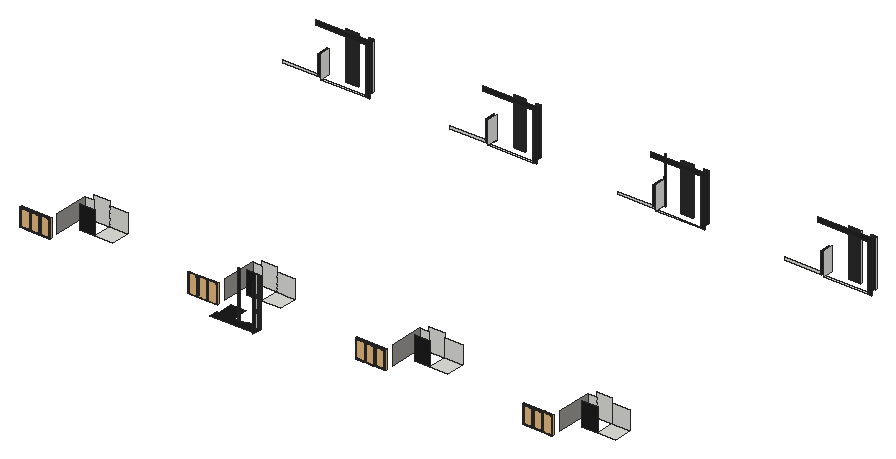
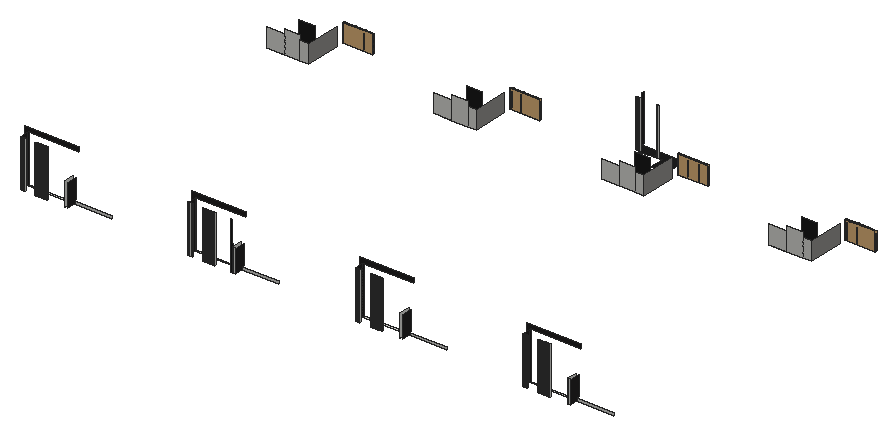
# SketchUp Ruby script. Lengths in inches.
U = 1.inch
M = Sketchup.active_model
def pt(a) = Geom::Point3d.new(a.map { |v| v * U })
def face(e, loops, mat)
  f = e.add_face(loops[0].map { |a| pt(a) })
  loops[1..].each { |l| e.add_face(l.map { |a| pt(a) }).erase! }
  f.material = f.back_material = mat if mat
  f
end
# faces: each face lists its corners as indices into pts; further lists are holes
def faces(e, pts, list, mat = nil) = list.each { |f| face(e, (f[0].is_a?(Array) ? f : [f]).map { |l| l.map { |i| pts[i] } }, mat) }
# xy, xz, yz: faces in a plane at the given z, y or x. An outline is a flat list of corners, or four numbers for a rectangle; further outlines are holes
def ring(l) = l.size == 4 ? [[l[0], l[1]], [l[2], l[1]], [l[2], l[3]], [l[0], l[3]]] : l.each_slice(2).to_a
def flat(e, list, mat, &to3) = list.each { |f| face(e, (f[0].is_a?(Array) ? f : [f]).map { |l| ring(l).map { |u, v| to3.(u, v) } }, mat) }
def xy(e, z, list, mat = nil) = flat(e, list, mat) { |x, y| [x, y, z] }
def xz(e, y, list, mat = nil) = flat(e, list, mat) { |x, z| [x, y, z] }
def yz(e, x, list, mat = nil) = flat(e, list, mat) { |y, z| [x, y, z] }
def lines(e, pts, list) = list.each { |a, b| e.add_line(pt(pts[a]), pt(pts[b])) }
# prism: a flat outline (further loops are holes) pulled along v
def prism(e, loops, v, mat = nil)
  f = face(e, loops, mat); d = Geom::Vector3d.new(v.map { |x| x * U })
  f.pushpull(f.normal.samedirection?(d) ? d.length : -d.length)
end
def box(e, o, s, mat = nil) = prism(e, [[o, [o[0] + s[0], o[1], o[2]], [o[0] + s[0], o[1] + s[1], o[2]], [o[0], o[1] + s[1], o[2]]]], [0, 0, s[2]], mat)
def at(x, y, z, deg = 0) = Geom::Transformation.translation(pt([x, y, z])) * Geom::Transformation.rotation(ORIGIN, Z_AXIS, deg.degrees)
def axes(o, x, y, z) = Geom::Transformation.new([*x, 0, *y, 0, *z, 0, *pt(o).to_a, 1])
def part(name) = M.definitions.add(name)
# library, detail: a bought-in or finely detailed component or shape, given as its bounding box
def library(name, o, s) = part(name).tap { |d| box(d.entities, o, s) }
def detail(e, o, s) = box(e.add_group.entities, o, s)
def put(e, d, t, mat = nil) = e.add_instance(d, t).tap { |i| i.material = mat if mat }
def group(e, t, mat = nil) = e.add_group.tap { |g| g.transformation = t; g.material = mat if mat }.entities
root = M.entities
M.materials.add("Wine2").color = [0, 0, 0]
M.materials["Wine2"].alpha = 0
M.materials.add("[0130_Gainsboro]").color = [39, 45, 50]
M.materials.add("[Color M08]").color = [30, 30, 30]
M.materials.add("[Field Square Tile]").color = [211, 167, 108]
M.materials.add("[Granite Dark Gray]").color = [38, 37, 37]
M.materials.add("[Granite Light Gray]").color = [149, 148, 144]
M.materials.add("[Slate]").color = [102, 110, 108]
c1 = part("Group\#55")
xy(c1.entities,0,[[0,-0.98,43.07,0],[0,0,43.07,1.4]],"[0130_Gainsboro]")
xy(c1.entities,0.3,[[0.3,-1.43,42.77,-0.98]],"[0130_Gainsboro]")
xy(c1.entities,2.95,[[2.95,-1.43,40.12,-0.63],[2.95,-0.63,40.12,0],[2.95,0,40.12,0.64],[2.95,0.64,40.12,1.4]],"[0130_Gainsboro]")
xy(c1.entities,3.54,[[3.54,-0.63,39.53,0],[3.54,0,39.53,0.64]],"[0130_Gainsboro]")
xy(c1.entities,111.8125,[[3.54,-0.63,39.53,0],[3.54,0,39.53,0.64]],"[0130_Gainsboro]")
xy(c1.entities,112.4,[[2.95,-1.43,40.12,-0.63],[2.95,-0.63,40.12,0],[2.95,0,40.12,0.64],[2.95,0.64,40.12,1.4]],"[0130_Gainsboro]")
xy(c1.entities,115.05,[[0.3,-1.43,42.77,-0.98]],"[0130_Gainsboro]")
xy(c1.entities,115.35,[[0,-0.98,43.07,0],[0,0,43.07,1.4]],"[0130_Gainsboro]")
xz(c1.entities,-1.43,[[[0.3,0.3,42.77,115.05],[2.95,2.95,40.12,112.4]]],"[0130_Gainsboro]")
xz(c1.entities,-0.98,[[[0,0,43.07,115.35],[0.3,0.3,42.77,115.05]]],"[0130_Gainsboro]")
xz(c1.entities,-0.63,[[[2.95,2.95,40.12,112.4],[3.54,3.54,39.53,111.8125]]],"[0130_Gainsboro]")
xz(c1.entities,0,[[3.54,3.54,39.53,111.8125]],"Wine2")
xz(c1.entities,0,[[[0,0,43.07,115.35],[2.95,2.95,40.12,112.4]],[[2.95,2.95,40.12,112.4],[3.54,3.54,39.53,111.8125]]],"[0130_Gainsboro]")
xz(c1.entities,0.64,[[[2.95,2.95,40.12,112.4],[3.54,3.54,39.53,111.8125]]],"[0130_Gainsboro]")
xz(c1.entities,1.4,[[[0,0,43.07,115.35],[2.95,2.95,40.12,112.4]]],"[0130_Gainsboro]")
yz(c1.entities,0,[[-0.98,0,0,115.35],[0,0,1.4,115.35]],"[0130_Gainsboro]")
yz(c1.entities,0.3,[[-1.43,0.3,-0.98,115.05]],"[0130_Gainsboro]")
yz(c1.entities,2.95,[[-1.43,2.95,-0.63,112.4],[-0.63,2.95,0,112.4],[0,2.95,0.64,112.4],[0.64,2.95,1.4,112.4]],"[0130_Gainsboro]")
yz(c1.entities,3.54,[[-0.63,3.54,0,111.8125],[0,3.54,0.64,111.8125]],"[0130_Gainsboro]")
yz(c1.entities,39.53,[[-0.63,3.54,0,111.8125],[0,3.54,0.64,111.8125]],"[0130_Gainsboro]")
yz(c1.entities,40.12,[[-1.43,2.95,-0.63,112.4],[-0.63,2.95,0,112.4],[0,2.95,0.64,112.4],[0.64,2.95,1.4,112.4]],"[0130_Gainsboro]")
yz(c1.entities,42.77,[[-1.43,0.3,-0.98,115.05]],"[0130_Gainsboro]")
yz(c1.entities,43.07,[[-0.98,0,0,115.35],[0,0,1.4,115.35]],"[0130_Gainsboro]")
c2 = part("Component\#21")
put(c2.entities,c1,axes([90.57,1.43,0],[1.05148,0,0],[0,1,0],[0,0,1]))
put(c2.entities,c1,axes([0,1.43,0],[1.05148,0,0],[0,1,0],[0,0,1]))
put(c2.entities,c1,axes([45.29,1.43,0],[1.05148,0,0],[0,1,0],[0,0,1]))
c3 = library("Curtains",[0,0,0],[121.73,8.19,117.22])
xy(root,134.5,[[1452.96,508.33,1458.38,511.08],[1551.31,508.33,1555.29,511.08],[534.46,697.21,629.77,792.52],[1413.21,697.21,1508.52,792.52],[2291.96,697.21,2387.27,792.52],
  [3170.71,697.21,3266.02,792.52],[442.35,2294.125,676.54,2294.125,676.54,2303.93,444.78,2303.93,444.78,2346.71,442.35,2346.71],[1321.1,2294.125,1555.29,2294.125,1555.29,2303.93,1323.53,2303.93,1323.53,2346.71,1321.1,2346.71],[2199.85,2294.125,2434.04,2294.125,2434.04,2303.93,2202.28,2303.93,2202.28,2346.71,2199.85,2346.71],[3078.6,2294.125,3312.79,2294.125,3312.79,2303.93,3081.03,2303.93,3081.03,2346.71,3078.6,2346.71],
  [534.46,2343.96,539.88,2346.71],[541.08,2343.96,546.51,2346.71],[547.71,2343.96,553.13,2346.71],[554.33,2343.96,559.76,2346.71],[560.96,2343.96,566.38,2346.71],
  [567.58,2343.96,573.01,2346.71],[574.21,2343.96,579.63,2346.71],[580.83,2343.96,586.26,2346.71],[587.46,2343.96,592.88,2346.71],[594.08,2343.96,599.51,2346.71],
  [653.06,2343.96,658.48,2346.71],[659.68,2343.96,665.11,2346.71],[666.31,2343.96,671.73,2346.71],[672.56,2343.96,676.54,2346.71],[676.54,2343.96,677.98,2346.71],
  [1413.21,2343.96,1418.63,2346.71],[1419.83,2343.96,1425.26,2346.71],[1426.46,2343.96,1431.88,2346.71],[1433.08,2343.96,1438.51,2346.71],[1439.71,2343.96,1445.13,2346.71],
  [1446.33,2343.96,1451.76,2346.71],[1452.96,2343.96,1458.38,2346.71],[1459.58,2343.96,1465.01,2346.71],[1466.21,2343.96,1471.63,2346.71],[1472.83,2343.96,1478.26,2346.71],
  [1531.81,2343.96,1537.23,2346.71],[1538.43,2343.96,1543.86,2346.71],[1545.06,2343.96,1550.48,2346.71],[1551.31,2343.96,1555.29,2346.71],[1555.29,2343.96,1556.73,2346.71],
  [2291.96,2343.96,2297.38,2346.71],[2298.58,2343.96,2304.01,2346.71],[2305.21,2343.96,2310.63,2346.71],[2311.83,2343.96,2317.26,2346.71],[2318.46,2343.96,2323.88,2346.71],
  [2325.08,2343.96,2330.51,2346.71],[2331.71,2343.96,2337.13,2346.71],[2338.33,2343.96,2343.76,2346.71],[2344.96,2343.96,2350.38,2346.71],[2351.58,2343.96,2357.01,2346.71],
  [2410.56,2343.96,2415.98,2346.71],[2417.18,2343.96,2422.61,2346.71],[2423.81,2343.96,2429.23,2346.71],[2430.06,2343.96,2434.04,2346.71],[2434.04,2343.96,2435.48,2346.71],
  [3170.71,2343.96,3176.13,2346.71],[3177.33,2343.96,3182.76,2346.71],[3183.96,2343.96,3189.38,2346.71],[3190.58,2343.96,3196.01,2346.71],[3197.21,2343.96,3202.63,2346.71],
  [3203.83,2343.96,3209.26,2346.71],[3210.46,2343.96,3215.88,2346.71],[3217.08,2343.96,3222.51,2346.71],[3223.71,2343.96,3229.13,2346.71],[3230.33,2343.96,3235.76,2346.71],
  [3289.31,2343.96,3294.73,2346.71],[3295.93,2343.96,3301.36,2346.71],[3302.56,2343.96,3307.98,2346.71],[3308.81,2343.96,3312.79,2346.71],[3312.79,2343.96,3314.23,2346.71]])
xy(root,134.5,[[1323.53,468.31,1555.29,468.31,1555.29,508.33,1551.31,508.33,1551.31,511.08,1550.48,511.08,1550.48,508.33,1545.06,508.33,1545.06,511.08,1543.86,511.08,1543.86,508.33,1538.43,508.33,1538.43,511.08,1537.23,511.08,1537.23,508.33,1531.81,508.33,1531.81,518.65,1483.9375,518.65,1483.9375,513.52,1478.26,513.52,1478.26,508.33,1472.83,508.33,1472.83,511.08,1471.63,511.08,1471.63,508.33,1466.21,508.33,1466.21,511.08,1465.01,511.08,1465.01,508.33,1459.58,508.33,1459.58,511.08,1458.38,511.08,1458.38,508.33,1452.96,508.33,1452.96,511.08,1451.76,511.08,1451.76,508.33,1446.33,508.33,1446.33,511.08,1445.13,511.08,1445.13,508.33,1439.71,508.33,1439.71,511.08,1438.51,511.08,1438.51,508.33,1433.08,508.33,1433.08,511.08,1431.88,511.08,1431.88,508.33,1426.46,508.33,1426.46,511.08,1425.26,511.08,1425.26,508.33,1419.83,508.33,1419.83,511.08,1418.63,511.08,1418.63,508.33,1413.21,508.33,1413.21,589.83,1332.45,589.83,1332.45,511.08,1323.53,511.08]],"[Color M08]")
xz(root,508.33,[[1551.31,134.5,1556.73,380.5]],"[Field Square Tile]")
xz(root,508.33,[[1439.71,134.5,1445.13,380.5],[1545.06,134.5,1550.48,380.5]],"[Granite Dark Gray]")
xz(root,511.08,[[1433.08,134.5,1438.51,380.5],[1531.81,134.5,1537.23,380.5],[1537.23,134.5,1538.43,380.5],[1538.43,134.5,1543.86,380.5]])
xz(root,697.21,[[453.7,134.5,534.46,254.5],[1332.45,134.5,1413.21,254.5],[2211.2,134.5,2291.96,254.5],[3089.95,134.5,3170.71,254.5]],"[Color M08]")
xz(root,792.52,[[406.85,134.5,453.7,231],[453.7,134.5,534.46,254.5],[534.46,134.5,629.77,231],[1285.6,134.5,1332.45,231],[1332.45,134.5,1413.21,254.5],
  [1413.21,134.5,1508.52,231],[2164.35,134.5,2211.2,231],[2211.2,134.5,2291.96,254.5],[2291.96,134.5,2387.27,231],[3043.1,134.5,3089.95,231],
  [3089.95,134.5,3170.71,254.5],[3170.71,134.5,3266.02,231]])
xz(root,2294.125,[[676.54,134.5,698.16,134.5,698.16,403.8125,414.98,403.8125,414.98,380.5,676.54,380.5],[1555.29,134.5,1576.91,134.5,1576.91,403.8125,1293.73,403.8125,1293.73,380.5,1555.29,380.5],[2434.04,134.5,2455.66,134.5,2455.66,403.8125,2172.48,403.8125,2172.48,380.5,2434.04,380.5],[3312.79,134.5,3334.41,134.5,3334.41,403.8125,3051.23,403.8125,3051.23,380.5,3312.79,380.5]],"[Granite Dark Gray]")
xz(root,2303.93,[[232.96,134.5,427.1,147.6875],[1111.71,134.5,1305.85,147.6875],[1990.46,134.5,2184.6,147.6875],[2869.21,134.5,3063.35,147.6875]])
xz(root,2343.96,[[672.56,134.5,677.98,380.5],[1551.31,134.5,1556.73,380.5],[2430.06,134.5,2435.48,380.5],[3308.81,134.5,3314.23,380.5]],"[Field Square Tile]")
xz(root,2343.96,[[534.46,134.5,539.88,380.5],[541.08,134.5,546.51,380.5],[547.71,134.5,553.13,380.5],[554.33,134.5,559.76,380.5],[560.96,134.5,566.38,380.5],
  [567.58,134.5,573.01,380.5],[574.21,134.5,579.63,380.5],[580.83,134.5,586.26,380.5],[587.46,134.5,592.88,380.5],[594.08,134.5,599.51,380.5],
  [653.06,134.5,658.48,380.5],[659.68,134.5,665.11,210.79],[666.31,134.5,671.73,380.5],[1413.21,134.5,1418.63,380.5],[1419.83,134.5,1425.26,380.5],
  [1426.46,134.5,1431.88,380.5],[1433.08,134.5,1438.51,380.5],[1439.71,134.5,1445.13,380.5],[1446.33,134.5,1451.76,380.5],[1452.96,134.5,1458.38,380.5],
  [1459.58,134.5,1465.01,380.5],[1466.21,134.5,1471.63,380.5],[1472.83,134.5,1478.26,380.5],[1531.81,134.5,1537.23,380.5],[1538.43,134.5,1543.86,210.79],
  [1545.06,134.5,1550.48,380.5],[2291.96,134.5,2297.38,380.5],[2298.58,134.5,2304.01,380.5],[2305.21,134.5,2310.63,380.5],[2311.83,134.5,2317.26,380.5],
  [2318.46,134.5,2323.88,380.5],[2325.08,134.5,2330.51,380.5],[2331.71,134.5,2337.13,380.5],[2338.33,134.5,2343.76,380.5],[2344.96,134.5,2350.38,380.5],
  [2351.58,134.5,2357.01,380.5],[2410.56,134.5,2415.98,380.5],[2417.18,134.5,2422.61,210.79],[2423.81,134.5,2429.23,380.5],[3170.71,134.5,3176.13,380.5],
  [3177.33,134.5,3182.76,380.5],[3183.96,134.5,3189.38,380.5],[3190.58,134.5,3196.01,380.5],[3197.21,134.5,3202.63,380.5],[3203.83,134.5,3209.26,380.5],
  [3210.46,134.5,3215.88,380.5],[3217.08,134.5,3222.51,380.5],[3223.71,134.5,3229.13,380.5],[3230.33,134.5,3235.76,380.5],[3289.31,134.5,3294.73,380.5],
  [3295.93,134.5,3301.36,210.79],[3302.56,134.5,3307.98,380.5]],"[Granite Dark Gray]")
xz(root,2346.71,[[427.1,134.5,442.35,134.5,442.35,254.5,433.97,254.5,433.97,251.5,427.1,251.5],[2184.6,134.5,2199.85,134.5,2199.85,254.5,2191.47,254.5,2191.47,251.5,2184.6,251.5],[2291.96,134.5,2297.38,380.5],[2297.38,134.5,2298.58,380.5],[2350.38,134.5,2351.58,380.5]])
xz(root,2346.71,[[2199.85,134.5,2211.2,134.5,2211.2,380.5,2202.28,380.5,2202.28,270.8125,2199.85,270.8125]],"[Color M08]")
yz(root,406.85,[[611.02,134.5,792.52,231]],"[Granite Light Gray]")
yz(root,427.1,[[2303.93,134.5,2303.93,147.6875,2294.125,147.6875,2294.125,251.5,2346.71,251.5,2346.71,134.5]],"[Granite Dark Gray]")
yz(root,442.35,[[2294.125,134.5,2346.71,254.5]])
yz(root,534.46,[[2343.96,134.5,2346.71,380.5]])
yz(root,539.88,[[2343.96,134.5,2346.71,380.5]])
yz(root,541.08,[[2343.96,134.5,2346.71,380.5]])
yz(root,546.51,[[2343.96,134.5,2346.71,380.5]])
yz(root,547.71,[[2343.96,134.5,2346.71,380.5]])
yz(root,553.13,[[2343.96,134.5,2346.71,380.5]])
yz(root,554.33,[[2343.96,134.5,2346.71,380.5]])
yz(root,559.76,[[2343.96,134.5,2346.71,380.5]])
yz(root,560.96,[[2343.96,134.5,2346.71,380.5]])
yz(root,566.38,[[2343.96,134.5,2346.71,380.5]])
yz(root,567.58,[[2343.96,134.5,2346.71,380.5]])
yz(root,573.01,[[2343.96,134.5,2346.71,380.5]])
yz(root,574.21,[[2343.96,134.5,2346.71,380.5]])
yz(root,579.63,[[2343.96,134.5,2346.71,380.5]])
yz(root,580.83,[[2343.96,134.5,2346.71,380.5]])
yz(root,586.26,[[2343.96,134.5,2346.71,380.5]])
yz(root,587.46,[[2343.96,134.5,2346.71,380.5]])
yz(root,592.88,[[2343.96,134.5,2346.71,380.5]])
yz(root,594.08,[[2343.96,134.5,2346.71,380.5]])
yz(root,599.51,[[2343.96,134.5,2346.71,380.5]])
yz(root,653.06,[[2343.96,134.5,2346.71,380.5]])
yz(root,658.48,[[2343.96,134.5,2346.71,380.5]])
yz(root,659.68,[[2343.96,134.5,2343.96,210.79,2337.02,210.79,2337.02,223.24,2343.96,223.24,2343.96,282.18,2337.02,282.18,2337.02,296.03,2343.96,296.03,2343.96,380.5,2346.71,380.5,2346.71,134.5]])
yz(root,665.11,[[2343.96,134.5,2346.71,134.5,2346.71,380.5,2343.96,380.5,2343.96,296.03,2337.02,296.03,2337.02,282.18,2343.96,282.18,2343.96,223.24,2337.02,223.24,2337.02,210.79,2343.96,210.79]])
yz(root,666.31,[[2343.96,134.5,2346.71,380.5]])
yz(root,671.73,[[2343.96,134.5,2346.71,380.5]])
yz(root,672.56,[[2343.96,134.5,2346.71,380.5]])
yz(root,676.54,[[2294.125,134.5,2303.93,380.5],[2303.93,134.5,2346.71,380.5]],"[Granite Dark Gray]")
yz(root,677.98,[[2343.96,134.5,2346.71,380.5]])
yz(root,1285.6,[[611.02,134.5,792.52,231]],"[Granite Light Gray]")
yz(root,1305.85,[[2303.93,134.5,2303.93,147.6875,2294.125,147.6875,2294.125,251.5,2346.71,251.5,2346.71,134.5]],"[Granite Dark Gray]")
yz(root,1321.1,[[2294.125,134.5,2346.71,254.5]])
yz(root,1413.21,[[2343.96,134.5,2346.71,380.5]])
yz(root,1418.63,[[2343.96,134.5,2346.71,380.5]])
yz(root,1419.83,[[2343.96,134.5,2346.71,380.5]])
yz(root,1425.26,[[2343.96,134.5,2346.71,380.5]])
yz(root,1426.46,[[2343.96,134.5,2346.71,380.5]])
yz(root,1431.88,[[2343.96,134.5,2346.71,380.5]])
yz(root,1433.08,[[2343.96,134.5,2346.71,380.5]])
yz(root,1438.51,[[2343.96,134.5,2346.71,380.5]])
yz(root,1439.71,[[2343.96,134.5,2346.71,380.5]])
yz(root,1445.13,[[2343.96,134.5,2346.71,380.5]])
yz(root,1446.33,[[2343.96,134.5,2346.71,380.5]])
yz(root,1451.76,[[2343.96,134.5,2346.71,380.5]])
yz(root,1452.96,[[2343.96,134.5,2346.71,380.5]])
yz(root,1458.38,[[2343.96,134.5,2346.71,380.5]])
yz(root,1459.58,[[2343.96,134.5,2346.71,380.5]])
yz(root,1465.01,[[2343.96,134.5,2346.71,380.5]])
yz(root,1466.21,[[2343.96,134.5,2346.71,380.5]])
yz(root,1471.63,[[2343.96,134.5,2346.71,380.5]])
yz(root,1472.83,[[2343.96,134.5,2346.71,380.5]])
yz(root,1478.26,[[2343.96,134.5,2346.71,380.5]])
yz(root,1531.81,[[508.33,134.5,511.08,380.5],[2343.96,134.5,2346.71,380.5]])
yz(root,1537.23,[[2343.96,134.5,2346.71,380.5]])
yz(root,1538.43,[[508.33,134.5,508.33,210.79,501.4,210.79,501.4,223.24,508.33,223.24,508.33,282.18,501.4,282.18,501.4,296.03,508.33,296.03,508.33,380.5,511.08,380.5,511.08,134.5],[2343.96,134.5,2343.96,210.79,2337.02,210.79,2337.02,223.24,2343.96,223.24,2343.96,282.18,2337.02,282.18,2337.02,296.03,2343.96,296.03,2343.96,380.5,2346.71,380.5,2346.71,134.5]])
yz(root,1543.86,[[508.33,134.5,511.08,134.5,511.08,380.5,508.33,380.5,508.33,296.03,501.4,296.03,501.4,282.18,508.33,282.18,508.33,223.24,501.4,223.24,501.4,210.79,508.33,210.79],[2343.96,134.5,2346.71,134.5,2346.71,380.5,2343.96,380.5,2343.96,296.03,2337.02,296.03,2337.02,282.18,2343.96,282.18,2343.96,223.24,2337.02,223.24,2337.02,210.79,2343.96,210.79]])
yz(root,1545.06,[[508.33,134.5,511.08,380.5],[2343.96,134.5,2346.71,380.5]])
yz(root,1550.48,[[508.33,134.5,511.08,380.5],[2343.96,134.5,2346.71,380.5]])
yz(root,1551.31,[[2343.96,134.5,2346.71,380.5]])
yz(root,1555.29,[[458.5,134.5,468.31,380.5],[2294.125,134.5,2303.93,380.5],[2303.93,134.5,2346.71,380.5]],"[Granite Dark Gray]")
yz(root,1556.73,[[2343.96,134.5,2346.71,380.5]])
yz(root,2164.35,[[611.02,134.5,792.52,231]],"[Granite Light Gray]")
yz(root,2184.6,[[2303.93,134.5,2303.93,147.6875,2294.125,147.6875,2294.125,251.5,2346.71,251.5,2346.71,134.5]],"[Granite Dark Gray]")
yz(root,2199.85,[[2294.125,134.5,2346.71,254.5]])
yz(root,2291.96,[[2343.96,134.5,2346.71,380.5]])
yz(root,2297.38,[[2343.96,134.5,2346.71,380.5]])
yz(root,2298.58,[[2343.96,134.5,2346.71,380.5]])
yz(root,2304.01,[[2343.96,134.5,2346.71,380.5]])
yz(root,2305.21,[[2343.96,134.5,2346.71,380.5]])
yz(root,2310.63,[[2343.96,134.5,2346.71,380.5]])
yz(root,2311.83,[[2343.96,134.5,2346.71,380.5]])
yz(root,2317.26,[[2343.96,134.5,2346.71,380.5]])
yz(root,2318.46,[[2343.96,134.5,2346.71,380.5]])
yz(root,2323.88,[[2343.96,134.5,2346.71,380.5]])
yz(root,2325.08,[[2343.96,134.5,2346.71,380.5]])
yz(root,2330.51,[[2343.96,134.5,2346.71,380.5]])
yz(root,2331.71,[[2343.96,134.5,2346.71,380.5]])
yz(root,2337.13,[[2343.96,134.5,2346.71,380.5]])
yz(root,2338.33,[[2343.96,134.5,2346.71,380.5]])
yz(root,2343.76,[[2343.96,134.5,2346.71,380.5]])
yz(root,2344.96,[[2343.96,134.5,2346.71,380.5]])
yz(root,2350.38,[[2343.96,134.5,2346.71,380.5]])
yz(root,2351.58,[[2343.96,134.5,2346.71,380.5]])
yz(root,2357.01,[[2343.96,134.5,2346.71,380.5]])
yz(root,2410.56,[[2343.96,134.5,2346.71,380.5]])
yz(root,2415.98,[[2343.96,134.5,2346.71,380.5]])
yz(root,2417.18,[[2343.96,134.5,2343.96,210.79,2337.02,210.79,2337.02,223.24,2343.96,223.24,2343.96,282.18,2337.02,282.18,2337.02,296.03,2343.96,296.03,2343.96,380.5,2346.71,380.5,2346.71,134.5]])
yz(root,2422.61,[[2343.96,134.5,2346.71,134.5,2346.71,380.5,2343.96,380.5,2343.96,296.03,2337.02,296.03,2337.02,282.18,2343.96,282.18,2343.96,223.24,2337.02,223.24,2337.02,210.79,2343.96,210.79]])
yz(root,2423.81,[[2343.96,134.5,2346.71,380.5]])
yz(root,2429.23,[[2343.96,134.5,2346.71,380.5]])
yz(root,2430.06,[[2343.96,134.5,2346.71,380.5]])
yz(root,2434.04,[[2294.125,134.5,2303.93,380.5],[2303.93,134.5,2346.71,380.5]],"[Granite Dark Gray]")
yz(root,2435.48,[[2343.96,134.5,2346.71,380.5]])
yz(root,3043.1,[[611.02,134.5,792.52,231]],"[Granite Light Gray]")
yz(root,3063.35,[[2303.93,134.5,2303.93,147.6875,2294.125,147.6875,2294.125,251.5,2346.71,251.5,2346.71,134.5]],"[Granite Dark Gray]")
yz(root,3078.6,[[2294.125,134.5,2346.71,254.5]])
yz(root,3170.71,[[2343.96,134.5,2346.71,380.5]])
yz(root,3176.13,[[2343.96,134.5,2346.71,380.5]])
yz(root,3177.33,[[2343.96,134.5,2346.71,380.5]])
yz(root,3182.76,[[2343.96,134.5,2346.71,380.5]])
yz(root,3183.96,[[2343.96,134.5,2346.71,380.5]])
yz(root,3189.38,[[2343.96,134.5,2346.71,380.5]])
yz(root,3190.58,[[2343.96,134.5,2346.71,380.5]])
yz(root,3196.01,[[2343.96,134.5,2346.71,380.5]])
yz(root,3197.21,[[2343.96,134.5,2346.71,380.5]])
yz(root,3202.63,[[2343.96,134.5,2346.71,380.5]])
yz(root,3203.83,[[2343.96,134.5,2346.71,380.5]])
yz(root,3209.26,[[2343.96,134.5,2346.71,380.5]])
yz(root,3210.46,[[2343.96,134.5,2346.71,380.5]])
yz(root,3215.88,[[2343.96,134.5,2346.71,380.5]])
yz(root,3217.08,[[2343.96,134.5,2346.71,380.5]])
yz(root,3222.51,[[2343.96,134.5,2346.71,380.5]])
yz(root,3223.71,[[2343.96,134.5,2346.71,380.5]])
yz(root,3229.13,[[2343.96,134.5,2346.71,380.5]])
yz(root,3230.33,[[2343.96,134.5,2346.71,380.5]])
yz(root,3235.76,[[2343.96,134.5,2346.71,380.5]])
yz(root,3289.31,[[2343.96,134.5,2346.71,380.5]])
yz(root,3294.73,[[2343.96,134.5,2346.71,380.5]])
yz(root,3295.93,[[2343.96,134.5,2343.96,210.79,2337.02,210.79,2337.02,223.24,2343.96,223.24,2343.96,282.18,2337.02,282.18,2337.02,296.03,2343.96,296.03,2343.96,380.5,2346.71,380.5,2346.71,134.5]])
yz(root,3301.36,[[2343.96,134.5,2346.71,134.5,2346.71,380.5,2343.96,380.5,2343.96,296.03,2337.02,296.03,2337.02,282.18,2343.96,282.18,2343.96,223.24,2337.02,223.24,2337.02,210.79,2343.96,210.79]])
yz(root,3302.56,[[2343.96,134.5,2346.71,380.5]])
yz(root,3307.98,[[2343.96,134.5,2346.71,380.5]])
yz(root,3308.81,[[2343.96,134.5,2346.71,380.5]])
yz(root,3312.79,[[2294.125,134.5,2303.93,380.5],[2303.93,134.5,2346.71,380.5]],"[Granite Dark Gray]")
yz(root,3314.23,[[2343.96,134.5,2346.71,380.5]])
put(root,c2,axes([2010.28,561.05,134.5],[1.13,0,0],[0,1,0],[0,0,0.83]))
put(root,c2,axes([2889.03,561.05,134.5],[1.13,0,0],[0,1,0],[0,0,0.83]))
put(root,c2,axes([252.78,561.05,134.5],[1.13,0,0],[0,1,0],[0,0,0.83]))
put(root,c2,axes([1131.53,561.05,134.5],[1.13,0,0],[0,1,0],[0,0,0.83]))
put(root,c3,axes([2010.28,561.05,134.75],[1.29555,0,0],[0,1,0],[0,0,0.8242]),"[Slate]")
put(root,c3,axes([2889.03,561.05,134.75],[1.29555,0,0],[0,1,0],[0,0,0.8242]),"[Slate]")
put(root,c3,axes([1131.53,561.05,134.75],[1.29555,0,0],[0,1,0],[0,0,0.8242]),"[Slate]")
put(root,c3,axes([252.78,561.05,134.75],[1.29555,0,0],[0,1,0],[0,0,0.8242]),"[Slate]")
